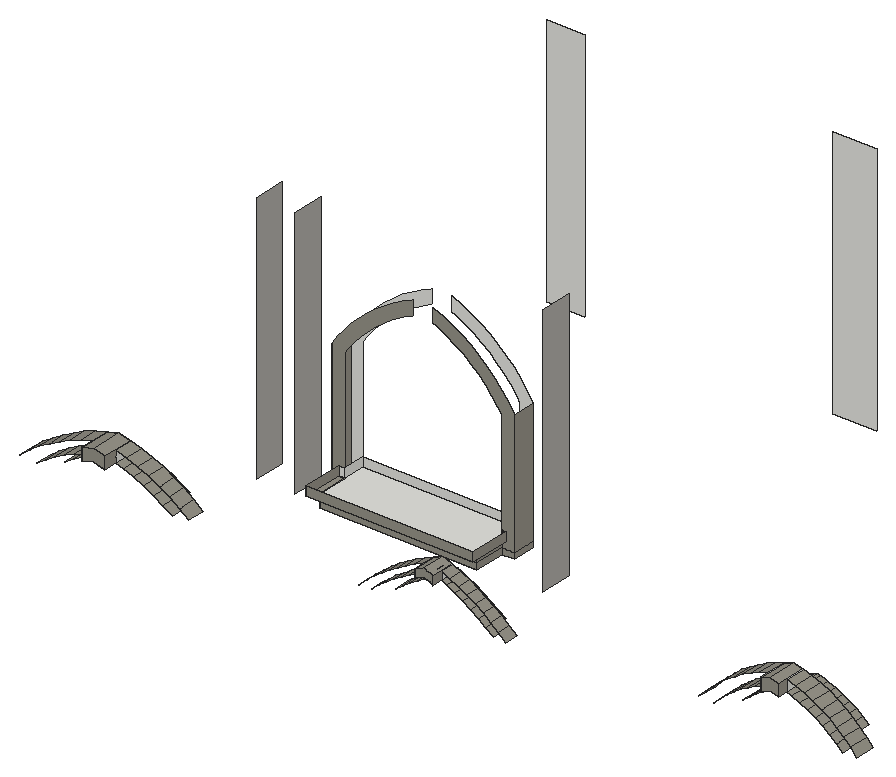
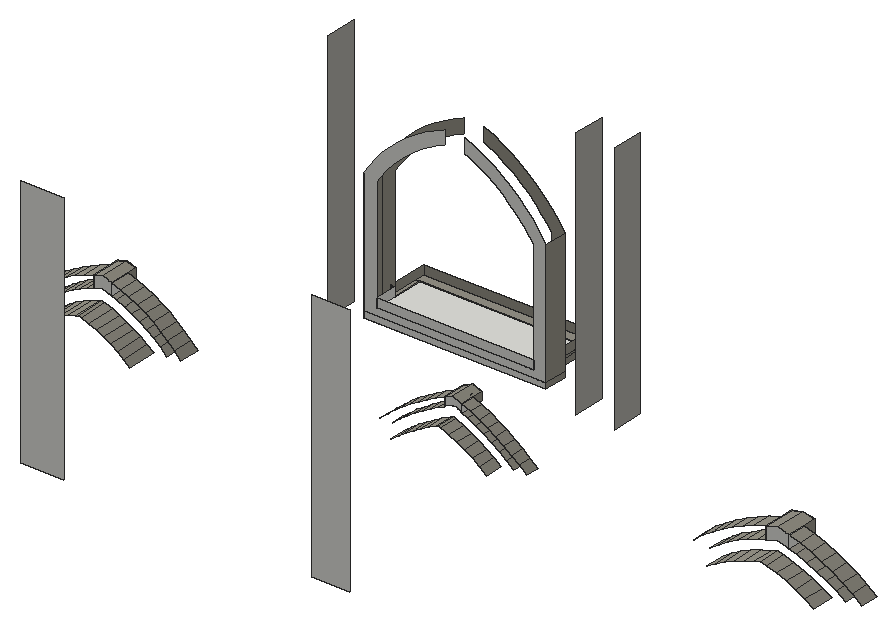
# SketchUp Ruby script. Lengths in inches.
U = 1.inch
M = Sketchup.active_model
def pt(a) = Geom::Point3d.new(a.map { |v| v * U })
def face(e, loops, mat)
  f = e.add_face(loops[0].map { |a| pt(a) })
  loops[1..].each { |l| e.add_face(l.map { |a| pt(a) }).erase! }
  f.material = f.back_material = mat if mat
  f
end
# faces: each face lists its corners as indices into pts; further lists are holes
def faces(e, pts, list, mat = nil) = list.each { |f| face(e, (f[0].is_a?(Array) ? f : [f]).map { |l| l.map { |i| pts[i] } }, mat) }
# xy, xz, yz: faces in a plane at the given z, y or x. An outline is a flat list of corners, or four numbers for a rectangle; further outlines are holes
def ring(l) = l.size == 4 ? [[l[0], l[1]], [l[2], l[1]], [l[2], l[3]], [l[0], l[3]]] : l.each_slice(2).to_a
def flat(e, list, mat, &to3) = list.each { |f| face(e, (f[0].is_a?(Array) ? f : [f]).map { |l| ring(l).map { |u, v| to3.(u, v) } }, mat) }
def xy(e, z, list, mat = nil) = flat(e, list, mat) { |x, y| [x, y, z] }
def xz(e, y, list, mat = nil) = flat(e, list, mat) { |x, z| [x, y, z] }
def yz(e, x, list, mat = nil) = flat(e, list, mat) { |y, z| [x, y, z] }
def lines(e, pts, list) = list.each { |a, b| e.add_line(pt(pts[a]), pt(pts[b])) }
# prism: a flat outline (further loops are holes) pulled along v
def prism(e, loops, v, mat = nil)
  f = face(e, loops, mat); d = Geom::Vector3d.new(v.map { |x| x * U })
  f.pushpull(f.normal.samedirection?(d) ? d.length : -d.length)
end
def box(e, o, s, mat = nil) = prism(e, [[o, [o[0] + s[0], o[1], o[2]], [o[0] + s[0], o[1] + s[1], o[2]], [o[0], o[1] + s[1], o[2]]]], [0, 0, s[2]], mat)
def at(x, y, z, deg = 0) = Geom::Transformation.translation(pt([x, y, z])) * Geom::Transformation.rotation(ORIGIN, Z_AXIS, deg.degrees)
def axes(o, x, y, z) = Geom::Transformation.new([*x, 0, *y, 0, *z, 0, *pt(o).to_a, 1])
def part(name) = M.definitions.add(name)
# library, detail: a bought-in or finely detailed component or shape, given as its bounding box
def library(name, o, s) = part(name).tap { |d| box(d.entities, o, s) }
def detail(e, o, s) = box(e.add_group.entities, o, s)
def put(e, d, t, mat = nil) = e.add_instance(d, t).tap { |i| i.material = mat if mat }
def group(e, t, mat = nil) = e.add_group.tap { |g| g.transformation = t; g.material = mat if mat }.entities
root = M.entities
M.materials.add("[Formica Graystone]").color = [149, 146, 135]
M.materials.add("[Terrazzo Tile Light]").color = [173, 171, 166]
xy(root,546.83,[[220.02,118.22,220.02,132.97,213.99,132.97,213.99,144.04,300.74,144.04,300.74,132.97,294.7,132.97,294.7,118.22]],"[Formica Graystone]")
xy(root,549.51,[[220.02,118.22,294.7,118.22,294.7,132.97,300.74,132.97,300.74,144.04,213.99,144.04,213.99,132.97,220.02,132.97]])
xy(root,553.04,[[220.02,118.22,294.7,144.04]])
xy(root,553.04,[[217.39,113.35,296.83,118.22],[217.39,118.22,220.02,132.97],[294.7,118.22,296.83,132.97]],"[Formica Graystone]")
xz(root,113.35,[[217.39,553.04,296.83,557.29]],"[Formica Graystone]")
xz(root,118.22,[[220.02,546.83,294.7,549.51],[220.02,549.51,294.7,553.04]],"[Formica Graystone]")
xz(root,128.85,[[98.39,519.51,99.875,519.97,103.87,520.9375,107.875,520,109.32,519.5625,109.32,525.375,103.85,526.66,98.39,525.34]],"[Formica Graystone]")
xz(root,132.41,[[262.4,522.42,262.4,526.6,258.18,528.37,253.91,526.7,253.91,522.5625,254.5,523.08,255.16,523.51,255.87,523.86,256.62,524.1,257.4,524.25,258.12,524.28,258.13,524.29,258.14,524.28,258.1875,524.29,258.97,524.22,259.74,524.05,260.48,523.78,261.18,523.41,261.83,522.96]],"[Formica Graystone]")
xz(root,132.97,[[217.39,553.04,220.02,557.29],[294.7,553.04,296.83,557.29]])
xz(root,132.97,[[213.99,546.83,220.02,549.51],[294.7,546.83,300.74,549.51],[213.99,549.51,220.02,549.51,220.02,553.04,217.39,553.04,217.39,557.29,220.02,557.29,220.02,606.39,221.74,608.86,224.67,612.57,227.82,616.09,231.17,619.43,234.72,622.55,238.44,625.46,242.33,628.15,246.38,630.6,250.5625,632.8,252.55,633.7,252.55,640.31,247.91,638.22,243.41,635.85,239.06,633.22,234.87,630.33,230.86,627.2,227.05,623.83,223.44,620.24,220.05,616.45,216.9,612.46,213.99,608.29],[294.7,549.51,300.74,549.51,300.74,608.39,297.92,612.65,294.83,616.72,291.49,620.58,287.9,624.22,284.07,627.61,280.04,630.74,275.81,633.61,271.4,636.1875,266.83,638.48,262.125,640.46,262.125,633.92,264.31,632.99,268.52,630.88,272.59,628.5,276.5,625.86,280.22,622.97,283.75,619.84,287.06,616.49,290.15,612.92,293,609.17,294.7,606.58,294.7,557.29,296.83,557.29,296.83,553.04,294.7,553.04]],"[Formica Graystone]")
xz(root,143.86,[[409.22,524.28,410.81,524.83,413.6,525.62,416.41,524.92,417.87,524.45,417.87,530.02,413.52,531.1,409.22,529.89]],"[Formica Graystone]")
xz(root,144.04,[[98.39,519.51,98.39,525.34,103.85,526.66,109.32,525.375,109.32,519.5625,107.875,520,103.87,520.9375,99.875,519.97],[262.4,522.42,261.83,522.96,261.18,523.41,260.48,523.78,259.74,524.05,258.97,524.22,258.1875,524.29,258.14,524.28,258.13,524.29,258.12,524.28,257.4,524.25,256.62,524.1,255.87,523.86,255.16,523.51,254.5,523.08,253.91,522.5625,253.91,526.7,258.18,528.37,262.4,526.6],[258.12,524.28,258.14,524.28,258.13,524.29],[213.99,546.83,300.74,549.51],[213.99,549.51,213.99,608.29,216.9,612.46,220.05,616.45,223.44,620.24,227.05,623.83,230.86,627.2,234.87,630.33,239.06,633.22,243.41,635.85,247.91,638.22,252.55,640.31,252.55,633.7,250.5625,632.8,246.38,630.6,242.33,628.15,238.44,625.46,234.72,622.55,231.17,619.43,227.82,616.09,224.67,612.57,221.74,608.86,220.02,606.39,220.02,553.04,294.7,553.04,294.7,606.58,293,609.17,290.15,612.92,287.06,616.49,283.75,619.84,280.22,622.97,276.5,625.86,272.59,628.5,268.52,630.88,264.31,632.99,262.125,633.92,262.125,640.46,266.83,638.48,271.4,636.1875,275.81,633.61,280.04,630.74,284.07,627.61,287.9,624.22,291.49,620.58,294.83,616.72,297.92,612.65,300.74,608.39,300.74,549.51],
  [220.02,553.04,294.7,557.29]])
xz(root,158.3,[[409.22,524.28,409.22,529.89,413.52,531.1,417.87,530.02,417.87,524.45,416.41,524.92,413.6,525.62,410.81,524.83]])
xz(root,301.14,[[181.54,540.875,199.67,660.875],[317.75,540.875,338.35,660.875]])
yz(root,98.39,[[135.41,519.51,144.04,525.34]])
yz(root,98.39,[[128.85,519.51,135.41,525.34]],"[Formica Graystone]")
yz(root,109.32,[[135.41,519.5625,144.04,525.375]])
yz(root,109.32,[[128.85,519.5625,135.41,525.375]],"[Formica Graystone]")
yz(root,181.54,[[128.91,540.875,144.04,660.875]],"[Terrazzo Tile Light]")
yz(root,199.67,[[128.91,540.875,144.04,660.875]],"[Terrazzo Tile Light]")
yz(root,213.99,[[132.97,546.83,144.04,549.51],[132.97,549.51,144.04,608.29]],"[Formica Graystone]")
yz(root,217.39,[[113.35,553.04,132.97,557.29]],"[Formica Graystone]")
yz(root,220.02,[[132.97,553.04,144.04,557.29]])
yz(root,220.02,[[118.22,546.83,132.97,549.51],[118.22,549.51,132.97,553.04]],"[Formica Graystone]")
yz(root,253.91,[[137.66,522.5625,144.04,526.7]])
yz(root,253.91,[[132.41,522.5625,137.66,526.7]],"[Formica Graystone]")
yz(root,262.4,[[137.66,522.42,144.04,526.6]])
yz(root,262.4,[[132.41,522.42,137.66,526.6]],"[Formica Graystone]")
yz(root,294.7,[[132.97,553.04,144.04,557.29]])
yz(root,294.7,[[118.22,546.83,132.97,549.51],[118.22,549.51,132.97,553.04]],"[Formica Graystone]")
yz(root,296.83,[[113.35,553.04,132.97,557.29]],"[Formica Graystone]")
yz(root,300.74,[[132.97,546.83,144.04,549.51],[132.97,549.51,144.04,608.39]],"[Formica Graystone]")
yz(root,317.75,[[128.91,540.875,144.04,660.875]],"[Terrazzo Tile Light]")
yz(root,409.22,[[148.68,524.28,158.3,529.89]])
yz(root,409.22,[[143.86,524.28,148.68,529.89]],"[Formica Graystone]")
yz(root,417.87,[[148.68,524.45,158.3,530.02]])
yz(root,417.87,[[143.86,524.45,148.68,530.02]],"[Formica Graystone]")
p = [[82.61,144.04,508.07],[78.34,144.04,505.48],[78.34,154.22,505.48],[82.61,154.22,508.07],[129.4375,144.04,505.6],[125.17,144.04,508.18],
  [125.17,154.22,508.18],[129.4375,154.22,505.6],[280.85,144.04,505.99],[277.45,144.04,508.52],[277.45,152.54,508.52],[280.85,152.54,505.99],
  [71.59,144.04,506.2],[75.92,144.04,509.2],[75.92,135.41,509.2],[71.59,135.41,506.2],[131.85,144.04,509.32],[136.18,144.04,506.32],
  [136.18,135.41,506.32],[131.85,135.41,509.32],[238.7,144.04,508.83],[235.32,144.04,506.31],[235.32,152.54,506.31],[238.7,152.54,508.83],
  [292.9375,144.04,506.65],[289.49,144.04,509.67],[289.49,137.66,509.67],[292.9375,137.66,506.65],[283.61,144.04,509.56],[287.06,144.04,506.78],
  [287.06,137.66,506.78],[283.61,137.66,509.56],[392.25,158.3,509.24],[389.35,158.3,506.76],[389.35,172.24,506.76],[392.25,172.24,509.24],
  [226.66,144.04,509.93],[223.25,144.04,506.87],[223.25,137.66,506.87],[226.66,137.66,509.93],[229.125,144.04,507.06],[232.54,144.04,509.86],
  [232.54,137.66,509.86],[229.125,137.66,507.06],[437.86,158.3,507.14],[435,158.3,509.62],[435,172.24,509.62],[437.86,172.24,507.14],
  [68.28,144.04,510.68],[63.87,144.04,507.2],[63.87,135.41,507.2],[68.28,135.41,510.68],[143.91,144.04,507.3],[139.5,144.04,510.79],
  [139.5,135.41,510.79],[143.91,135.41,507.3],[382.95,158.3,507.66],[385.92,158.3,510.53],[385.92,148.68,510.53],[382.95,148.68,507.66],
  [441.33,158.3,510.88],[444.25,158.3,507.97],[444.25,148.68,507.97],[441.33,148.68,510.88],[87.04,144.04,510.4],[87.04,154.22,510.4],
  [379.15,158.3,511.35],[376.14,158.3,508.06],[376.14,148.68,508.06],[379.15,148.68,511.35],[120.74,144.04,510.5],[120.74,154.22,510.5],
  [451.07,158.3,508.24],[448.12,158.3,511.6],[448.12,148.68,511.6],[451.07,148.68,508.24],[273.94,144.04,510.92],[273.94,152.54,510.92],
  [242.1875,144.04,511.2],[242.1875,152.54,511.2],[80.43,144.04,511.9375],[80.43,135.41,511.9375],[395.3,158.3,511.53],[395.3,172.24,511.53],
  [127.35,144.04,512.05],[127.35,135.41,512.05],[280.0625,144.04,512.2],[280.0625,137.66,512.2],[431.99,158.3,511.9],[431.99,172.24,511.9],
  [285.93,144.04,512.55],[285.93,137.66,512.55],[230.21,144.04,512.84],[230.21,137.66,512.84],[236.08,144.04,512.5],[236.08,137.66,512.5],
  [91.6,144.04,512.45],[91.6,154.22,512.45],[116.18,144.04,512.53],[116.18,154.22,512.53],[389.0625,158.3,513.22],[389.0625,148.68,513.22],
  [72.89,144.04,513.875],[72.89,135.41,513.875],[134.89,144.04,513.99],[134.89,135.41,513.99],[270.34,144.04,513.16],[270.34,152.54,513.16],
  [438.22,158.3,513.58],[438.22,148.68,513.58],[245.78,144.04,513.41],[245.78,152.54,513.41],[382.35,158.3,514.45],[382.35,148.68,514.45],
  [398.49,158.3,513.64],[398.49,172.24,513.64],[444.94,158.3,514.76],[444.94,148.68,514.76],[85.1,144.04,514.39],[85.1,135.41,514.39],
  [428.83,158.3,513.97],[428.83,172.24,513.97],[122.67,144.04,514.49],[122.67,135.41,514.49],[276.41,144.04,514.69],[276.41,137.66,514.69],
  [96.28,144.04,514.21],[96.28,154.22,514.21],[239.74,144.04,514.99],[239.74,137.66,514.99],[282.26,144.04,515.28],[282.26,137.66,515.28],
  [111.5,144.04,514.27],[111.5,154.22,514.27],[233.89,144.04,515.59],[233.89,137.66,515.59],[266.65,144.04,515.27],[266.65,152.54,515.27],
  [392.36,158.3,515.7],[392.36,148.68,515.7],[249.47,144.04,515.46],[249.47,152.54,515.46],[434.93,158.3,516.07],[434.93,148.68,516.07],
  [401.8,158.3,515.54],[401.8,172.24,515.54],[77.69,144.04,516.79],[77.69,135.41,516.79],[130.08,144.04,516.9],[130.08,135.41,516.9],
  [425.54,158.3,515.83],[425.54,172.24,515.83],[101.05,144.04,515.6875],[101.05,154.22,515.6875],[106.73,144.04,515.71],[106.73,154.22,515.71],
  [89.91,144.04,516.55],[89.91,135.41,516.55],[117.86,144.04,516.64],[117.86,135.41,516.64],[385.74,158.3,517.35],[385.74,148.68,517.35],
  [272.65,144.04,517.04],[272.65,137.66,517.04],[441.56,158.3,517.7],[441.56,148.68,517.7],[243.5,144.04,517.3],[243.5,137.66,517.3],
  [278.48,144.04,517.86],[278.48,137.66,517.86],[262.89,144.04,517.22],[262.89,152.54,517.22],[253.24,144.04,517.33],[253.24,152.54,517.33],
  [405.22,158.3,517.23],[405.22,172.24,517.23],[237.68,144.04,518.16],[237.68,137.66,518.16],[103.89,144.04,516.375],[103.89,154.22,516.375],
  [105.93,154.22,515.9],[395.8125,158.3,517.98],[395.8125,148.68,517.98],[422.13,158.3,517.46],[422.13,172.24,517.46],[431.48,158.3,518.33],
  [431.48,148.68,518.33],[94.84,144.04,518.41],[94.84,135.41,518.41],[112.92,144.04,518.47],[112.92,135.41,518.47],[82.66,144.04,519.4],
  [82.66,135.41,519.4],[125.1,144.04,519.51],[125.1,135.41,519.51],[268.81,144.04,519.23],[268.81,137.66,519.23],[259.04,144.04,519.01],
  [259.04,152.54,519.01],[260.125,152.54,518.51],[408.74,158.3,518.71],[408.74,172.24,518.71],[247.37,144.04,519.45],[247.37,137.66,519.45],
  [257.1,144.04,519.04],[255.17,152.54,518.1875],[257.1,152.54,519.04],[389.31,158.3,520.03],[389.31,148.68,520.03],[418.61,158.3,518.85],
  [418.61,172.24,518.85],[437.99,158.3,520.4],[437.99,148.68,520.4],[274.59,144.04,520.28],[274.59,137.66,520.28],[399.4,158.3,520.04],
  [399.4,148.68,520.04],[241.59,144.04,520.57],[241.59,137.66,520.57],[427.89,158.3,520.36],[427.89,148.68,520.36],[98.39,144.04,519.51],
  [98.39,135.41,519.51],[109.32,144.04,519.5625],[109.32,135.41,519.5625],[412.35,158.3,519.97],[412.35,172.24,519.97],[415.02,158.3,520.01],
  [415.02,172.24,520.01],[416.87,172.24,519.42],[258.07,144.04,519.42],[258.07,152.54,519.42],[258.8125,152.54,519.11],[264.88,144.04,521.26],
  [264.88,137.66,521.26],[87.78,144.04,521.7],[87.78,135.41,521.7],[251.32,144.04,521.42],[251.32,137.66,521.42],[99.875,144.04,519.97],
  [99.875,128.85,519.97],[98.39,128.85,519.51],[119.96,144.04,521.79],[119.96,135.41,521.79],[107.875,144.04,520],[109.32,128.85,519.5625],
  [107.875,128.85,520],[103.87,144.04,520.9375],[103.87,128.85,520.9375],[393.03,158.3,522.49],[393.03,148.68,522.49],[403.1,158.3,521.87],
  [403.1,148.68,521.87],[413.68,158.3,520.34],[413.68,172.24,520.34],[270.62,144.04,522.55],[270.62,137.66,522.55],[424.17,158.3,522.13],
  [424.17,148.68,522.13],[434.24,158.3,522.86],[434.24,148.68,522.86],[245.6,144.04,522.8],[245.6,137.66,522.8],[262.4,144.04,522.42],
  [262.4,137.66,522.42],[253.91,144.04,522.5625],[253.91,137.66,522.5625],[93.03,144.04,523.68],[93.03,135.41,523.68],[114.7,144.04,523.75],
  [114.7,135.41,523.75],[406.91,158.3,523.47],[406.91,148.68,523.47],[420.34,158.3,523.66],[420.34,148.68,523.66],[261.83,144.04,522.96],
  [262.4,132.41,522.42],[261.83,132.41,522.96],[396.9,158.3,524.71],[396.9,148.68,524.71],[254.5,144.04,523.08],[254.5,132.41,523.08],
  [253.91,132.41,522.5625],[266.55,144.04,524.66],[266.55,137.66,524.66],[249.71,144.04,524.84],[249.71,137.66,524.84],[430.34,158.3,525.06],
  [430.34,148.68,525.06],[261.18,144.04,523.41],[261.18,132.41,523.41],[255.16,144.04,523.51],[255.16,132.41,523.51],[260.48,144.04,523.78],
  [260.48,132.41,523.78],[255.87,144.04,523.86],[255.87,132.41,523.86],[409.22,158.3,524.28],[409.22,148.68,524.28],[98.39,144.04,525.34],
  [98.39,135.41,525.34],[417.87,158.3,524.45],[417.87,148.68,524.45],[259.74,144.04,524.05],[259.74,132.41,524.05],[109.32,144.04,525.375],
  [109.32,135.41,525.375],[256.62,144.04,524.1],[256.62,132.41,524.1],[257.4,144.04,524.25],[257.4,132.41,524.25],[258.97,144.04,524.22],
  [258.97,132.41,524.22],[258.12,144.04,524.28],[258.12,132.41,524.28],[258.1875,144.04,524.29],[258.1875,132.41,524.29],[258.13,144.04,524.29],
  [258.13,132.41,524.29],[258.14,144.04,524.28],[258.14,132.41,524.28],[410.81,158.3,524.83],[410.81,143.86,524.83],[409.22,143.86,524.28],
  [416.41,158.3,524.92],[417.87,143.86,524.45],[416.41,143.86,524.92],[262.4,144.04,526.6],[262.4,137.66,526.6],[400.9,158.3,526.69],
  [400.9,148.68,526.69],[253.91,144.04,526.7],[253.91,137.66,526.7],[413.6,158.3,525.62],[413.6,143.86,525.62],[426.29,158.3,526.99],
  [426.29,148.68,526.99],[103.85,144.04,526.66],[98.39,128.85,525.34],[103.85,128.85,526.66],[109.32,128.85,525.375],[258.18,144.04,528.37],
  [258.18,132.41,528.37],[262.4,132.41,526.6],[253.91,132.41,526.7],[405.01,158.3,528.42],[405.01,148.68,528.42],[422.13,158.3,528.65],
  [422.13,148.68,528.65],[409.22,158.3,529.89],[409.22,148.68,529.89],[417.87,158.3,530.02],[417.87,148.68,530.02],[413.52,158.3,531.1],
  [409.22,143.86,529.89],[413.52,143.86,531.1],[417.87,143.86,530.02],[109.32,144.04,519.51]]
faces(root,p,[[0,1,2,3],[4,5,6,7],[8,9,10,11],[12,13,14,15],[16,17,18,19],[20,21,22,23],[24,25,26,27],[28,29,30,31],
  [32,33,34,35],[36,37,38,39],[40,41,42,43],[44,45,46,47],[48,49,50,51],[52,53,54,55],[56,57,58,59],[60,61,62,63],
  [64,0,3,65],[66,67,68,69],[5,70,71,6],[72,73,74,75],[9,76,77,10],[78,20,23,79],[13,80,81,14],[82,32,35,83],
  [84,16,19,85],[86,28,31,87],[45,88,89,46],[25,90,91,26],[92,36,39,93],[41,94,95,42],[96,64,65,97],[70,98,99,71],
  [57,100,101,58],[102,48,51,103],[53,104,105,54],[76,106,107,77],[108,60,63,109],[110,78,79,111],[112,66,69,113],[114,82,83,115],
  [73,116,117,74],[80,118,119,81],[88,120,121,89],[122,84,85,123],[124,86,87,125],[126,96,97,127],[94,128,129,95],[90,130,131,91],
  [98,132,133,99],[134,92,93,135],[106,136,137,107],[100,138,139,101],[140,110,111,141],[142,108,109,143],[144,114,115,145],[146,102,103,147],
  [104,148,149,105],[120,150,151,121],[152,126,127,153],[132,154,155,133],[118,156,157,119],[158,122,123,159],[160,112,113,161],[162,124,125,163],
  [116,164,165,117],[128,166,167,129],[130,168,169,131],[136,170,171,137],[172,140,141,173],[174,144,145,175],[176,134,135,177],[178,152,153,179],
  [154,178,179,180,155],[138,181,182,139],[150,183,184,151],[185,142,143,186],[156,187,188,157],[189,158,159,190],[191,146,147,192],[148,193,194,149],
  [195,162,163,196],[170,197,198,199,171],[200,174,175,201],[166,202,203,167],[204,172,173,205,206],[207,160,161,208],[183,209,210,184],[164,211,212,165],
  [168,213,214,169],[181,215,216,182],[217,176,177,218],[219,185,186,220],[187,221,222,188],[223,189,190,224],[225,200,201,226],[209,227,228,229,210],
  [230,204,206,231],[197,230,231,232,198],[233,195,196,234],[235,191,192,236],[202,237,238,203],[221,239,240,241,222],[193,242,243,194],[244,223,224,245,246],
  [239,247,248,240],[247,244,246,248],[249,207,208,250],[215,251,252,216],[253,225,226,254],[227,253,254,228],[213,255,256,214],[257,219,220,258],
  [211,259,260,212],[261,217,218,262],[263,233,234,264],[237,265,266,238],[267,235,236,268],[242,269,270,243],[251,271,272,252],[273,257,258,274],
  [275,263,264,276,277],[278,249,250,279],[265,280,281,282,266],[255,283,284,256],[285,261,262,286],[259,287,288,260],[289,275,277,290],[280,291,292,281],
  [293,289,290,294],[291,295,296,292],[271,297,298,272],[299,267,268,300],[301,273,274,302],[303,293,294,304],[269,305,306,270],[295,307,308,296],
  [307,309,310,308],[311,303,304,312],[309,313,314,310],[315,311,312,316],[319,315,316,320],[297,321,322,323,298],[324,301,302,325,326],[283,327,328,284],
  [329,278,279,330],[331,285,286,332],[321,333,334,322],[333,324,326,334],[287,335,336,288],[337,299,300,338,339],[305,337,339,340,306],[327,341,342,343,328],
  [341,331,332,344,342],[345,329,330,346],[335,347,348,336],[349,345,346,350],[347,351,352,348],[353,349,350,354,355],[351,353,355,356,352]],"[Formica Graystone]")
faces(root,p,[[313,317,318,314],[317,319,320,318]])
lines(root,p,[[223,357]])
